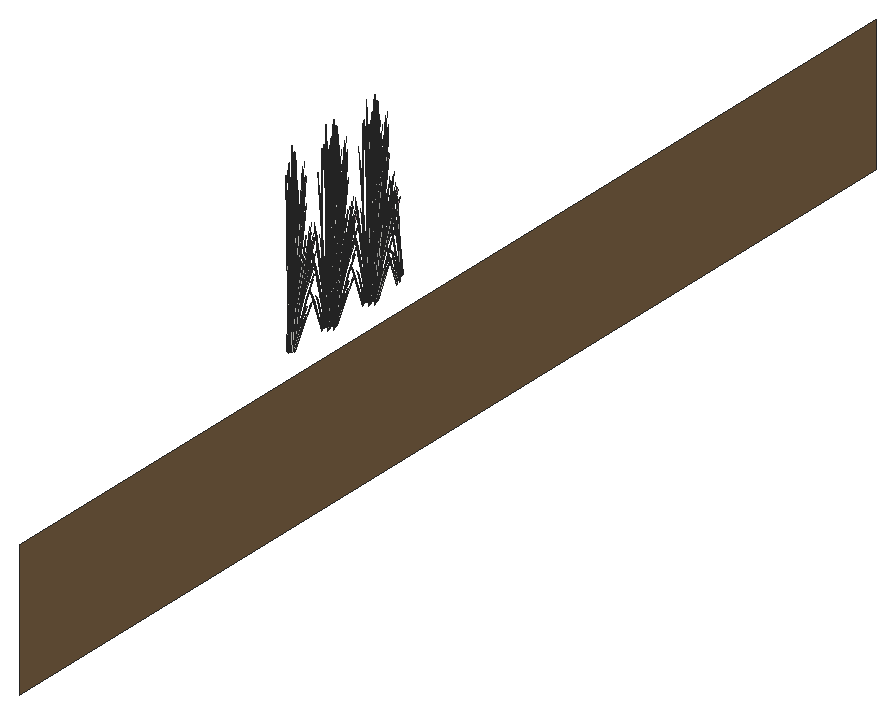
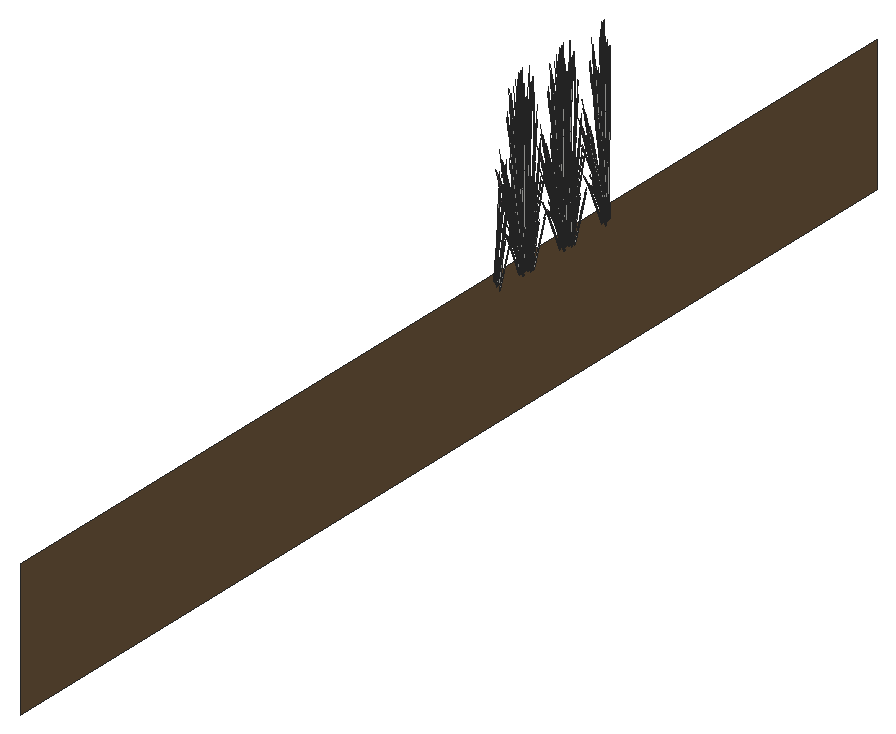
# SketchUp Ruby script. Lengths in inches.
U = 1.inch
M = Sketchup.active_model
def pt(a) = Geom::Point3d.new(a.map { |v| v * U })
def face(e, loops, mat)
  f = e.add_face(loops[0].map { |a| pt(a) })
  loops[1..].each { |l| e.add_face(l.map { |a| pt(a) }).erase! }
  f.material = f.back_material = mat if mat
  f
end
# faces: each face lists its corners as indices into pts; further lists are holes
def faces(e, pts, list, mat = nil) = list.each { |f| face(e, (f[0].is_a?(Array) ? f : [f]).map { |l| l.map { |i| pts[i] } }, mat) }
# xy, xz, yz: faces in a plane at the given z, y or x. An outline is a flat list of corners, or four numbers for a rectangle; further outlines are holes
def ring(l) = l.size == 4 ? [[l[0], l[1]], [l[2], l[1]], [l[2], l[3]], [l[0], l[3]]] : l.each_slice(2).to_a
def flat(e, list, mat, &to3) = list.each { |f| face(e, (f[0].is_a?(Array) ? f : [f]).map { |l| ring(l).map { |u, v| to3.(u, v) } }, mat) }
def xy(e, z, list, mat = nil) = flat(e, list, mat) { |x, y| [x, y, z] }
def xz(e, y, list, mat = nil) = flat(e, list, mat) { |x, z| [x, y, z] }
def yz(e, x, list, mat = nil) = flat(e, list, mat) { |y, z| [x, y, z] }
def lines(e, pts, list) = list.each { |a, b| e.add_line(pt(pts[a]), pt(pts[b])) }
# prism: a flat outline (further loops are holes) pulled along v
def prism(e, loops, v, mat = nil)
  f = face(e, loops, mat); d = Geom::Vector3d.new(v.map { |x| x * U })
  f.pushpull(f.normal.samedirection?(d) ? d.length : -d.length)
end
def box(e, o, s, mat = nil) = prism(e, [[o, [o[0] + s[0], o[1], o[2]], [o[0] + s[0], o[1] + s[1], o[2]], [o[0], o[1] + s[1], o[2]]]], [0, 0, s[2]], mat)
def at(x, y, z, deg = 0) = Geom::Transformation.translation(pt([x, y, z])) * Geom::Transformation.rotation(ORIGIN, Z_AXIS, deg.degrees)
def axes(o, x, y, z) = Geom::Transformation.new([*x, 0, *y, 0, *z, 0, *pt(o).to_a, 1])
def part(name) = M.definitions.add(name)
# library, detail: a bought-in or finely detailed component or shape, given as its bounding box
def library(name, o, s) = part(name).tap { |d| box(d.entities, o, s) }
def detail(e, o, s) = box(e.add_group.entities, o, s)
def put(e, d, t, mat = nil) = e.add_instance(d, t).tap { |i| i.material = mat if mat }
def group(e, t, mat = nil) = e.add_group.tap { |g| g.transformation = t; g.material = mat if mat }.entities
root = M.entities
M.materials.add("LightPink_Translucent").color = [144, 107, 117]
M.materials["LightPink_Translucent"].alpha = 0.75
M.materials.add("Soil_03_1K").color = [122, 96, 67]
c1 = part("blade")
p = [[2.15,0.21,22],[0,0.17,0],[0.09,0.45,0],[2.18,0.31,22],[2.29,0.31,22],[0.38,0.45,0],
  [2.48,0.24,33],[2.49,0.24,33],[2.48,0.22,33]]
faces(c1.entities,p,[[0,1,2,3],[4,5,2,3],[6,3,4,7],[8,0,3,6]])
c2 = part("seeds")
p = [[0.3,-0.1,1.38],[-0.01,-0.03,1.59],[-0.01,-0.03,0.03],[0.14,-0.07,-0.07],[0.29,-0.03,3],[0.15,0.01,3.11]]
faces(c2.entities,p,[[0,1,2,3],[1,0,4,5]],"LightPink_Translucent")
c3 = part("blade with seeds")
put(c3.entities,c1,at(0,0,0))
put(c3.entities,c2,axes([2.4,0.25,30.99],[1.5799,-0.05474,1.17369],[-0.12525,1.92788,0.29478],[-0.07173,-0.02425,1.56792]))
yz(root,410.57,[[509.26,-48,890.67,0]],"Soil_03_1K")
put(root,c3,axes([402.5,638.32,2.38],[-0.44609,-0.09826,0.49198],[0.09078,-0.55493,0.19306],[0.06519,0.05359,1.70813]))
put(root,c3,axes([402.15,639.6875,2.2],[-0.11516,-0.40207,0],[0.32884,-0.1408,0],[0,0,1.54371]))
put(root,c3,axes([402.58,639.63,2.18],[0.37054,-0.15823,-0.19198],[0.1302,0.45581,0.00008],[0.0409,-0.01749,1.73897]))
put(root,c3,axes([402.62,638.77,2.21],[0.24637,0.30123,0],[-0.24637,0.30123,0],[0,0,1.69266]))
put(root,c3,axes([403.29,638.64,2.47],[-0.2773,-0.3397,0.17642],[0.27945,-0.32949,0.35086],[-0.03063,0.06937,1.60407]))
put(root,c3,axes([402.78,638.125,2.06],[0.36714,0.07646,-0.62353],[-0.07747,0.47163,-0.16365],[0.10956,0.05715,1.37633]))
put(root,c3,axes([404.4,638.95,2.77],[-0.21807,0.07699,1.1486],[0.10265,-0.31819,0.84392],[0.11568,0.02177,0.25299]))
put(root,c3,axes([402.62,638.42,2.72],[0.17124,-0.42022,0.44739],[0.35581,0.20224,-0.21531],[0,0.09687,1.43643]))
put(root,c3,axes([402.55,638.66,2.29],[0,0.53934,-0.05637],[-0.44133,0,0],[0,0.01695,1.79368]))
put(root,c3,axes([402.58,638.28,2.21],[0.21202,0.39143,-0.44739],[-0.32115,0.27564,0.21531],[0.06861,0.04843,1.43643]))
put(root,c3,axes([404.02,639.93,3.93],[-0.06755,-0.39203,-0.03492],[0.31928,-0.09013,-0.15832],[0.06667,0.02485,0.52218]))
put(root,c3,axes([403.52,638.65,2.48],[0,-0.46636,0.49651],[0.39487,0,0],[0,0.10622,1.57504]))
put(root,c3,axes([402.77,638.51,2.62],[0.32884,-0.136,0.1448],[0.11516,0.38837,-0.41347],[0,0.08547,1.26744]))
put(root,c3,axes([403.99,639.46,2.59],[-0.085,-0.1147,1.43002],[0.1106,-0.37943,-0.30754],[0.17198,0.0514,0.61141]))
put(root,c3,axes([402.47,639.88,2.2],[0.35581,0.20937,0],[-0.17124,0.43505,0],[0,0,1.74954]))
put(root,c3,axes([403.21,639.69,4.98],[0.35281,0.01123,-0.71045],[-0.0237,0.47284,0.08574],[0.14947,0.0499,1.00501]))
put(root,c3,axes([402.8125,640.07,2.48],[0.33032,-0.23318,0.49651],[0.19744,0.41812,0],[-0.07523,0.05311,1.57504]))
put(root,c3,axes([402.34,639.7,2.29],[0.15345,0.53576,-0.06012],[-0.43845,0.18773,0],[0.00536,0.01871,1.72173]))
put(root,c3,axes([403.78,638.73,2.375],[0.44133,0,0],[0,0.52122,-0.51607],[0,0.11871,1.63711]))
put(root,c3,axes([403.61,639,2.2],[-0.44111,-0.00373,-0.04976],[0,-0.52122,0.49943],[-0.01386,0.11865,1.58352]))
put(root,c3,axes([402.65,638.55,2.67],[0.39748,0.22252,-0.29095],[-0.19139,0.46966,-0.50002],[0.01249,0.11531,1.59708]))
put(root,c3,axes([403.42,639.89,4.53],[0.20082,0.29199,-0.35414],[-0.2293,0.2764,0.4572],[0.1165,0.04206,0.87481]))
put(root,c3,axes([403.52,639.08,2.03],[-0.24637,0.29097,-0.30978],[-0.24637,-0.29097,0.30978],[0,0.09372,1.38974]))
put(root,c3,axes([402.61,638.9,2.21],[-0.17124,0.42022,-0.44739],[-0.35581,-0.20224,0.21531],[0,0.09687,1.43643]))
put(root,c3,axes([402.62,640.1,2.33],[0.44186,0.15158,0.30756],[-0.11054,0.54181,-0.36492],[-0.07313,0.06781,1.64885]))
put(root,c3,axes([403.6875,639.09,2.02],[0,0.46636,-0.49651],[-0.39487,0,0],[0,0.10622,1.57504]))
put(root,c3,axes([402.7,639.14,3.875],[-0.1311,-0.08035,1.71376],[0.27131,-0.33708,0.13857],[0.16909,0.15206,0.73262]))
put(root,c3,axes([403.18,640.05,2.77],[-0.19872,-0.13409,1.1486],[0.2566,-0.13625,0.84392],[0.06921,0.11541,0.25299]))
put(root,c3,axes([403.24,640.55,1.49],[0.02571,-0.06733,1.76342],[0.32373,-0.19829,-0.26939],[0.09815,0.10263,0.30037]))
put(root,c3,axes([402.8125,639.02,2.09],[0.12941,0.42699,-0.69212],[-0.37279,0.15378,-0.18165],[0.0143,0.14459,1.52773]))
put(root,c3,axes([402.74,640.24,4.68],[0.34827,-0.11086,-0.51099],[0.06092,0.41983,-0.3958],[0.09354,0.12031,0.97773]))
put(root,c3,axes([403.22,640.66,2.67],[-0.22633,-0.01463,1.0506],[0.14947,-0.31064,0.58006],[0.08941,0.11036,0.8241]))
put(root,c3,axes([402.48,639.91,2.59],[0.00623,-0.15459,1.43002],[0.29764,-0.17268,-0.30754],[0.09188,0.18503,0.61141]))
put(root,c3,axes([401.73,640.54,1.49],[0.05712,-0.02538,1.76342],[0.34359,0.13968,-0.26939],[0.01005,0.15742,0.30037]))
put(root,c3,axes([401.96,640.43,4.68],[0.34695,0.11691,-0.51099],[-0.11892,0.40083,-0.3958],[0.03181,0.16138,0.97773]))
put(root,c3,axes([402.16,639.61,3.875],[-0.08068,-0.14973,1.71376],[0.3728,-0.12606,0.13857],[0.08426,0.23506,0.73262]))
put(root,c3,axes([401.8,640.68,4.53],[-0.1064,0.35863,-0.35414],[-0.31043,-0.1046,0.4572],[0.02846,0.14439,0.87481]))
put(root,c3,axes([401.84,640.36,4.98],[0.16845,0.3792,-0.71045],[-0.34676,0.21133,0.08574],[0.03939,0.18322,1.00501]))
put(root,c3,axes([402.72,655.13,2.59],[-0.10032,0.0944,1.43002],[-0.30046,-0.16522,-0.30754],[0.05569,-0.20547,0.61141]))
put(root,c3,axes([401.98,654.62,1.49],[-0.0592,0.0168,1.76342],[-0.32738,-0.18913,-0.26939],[0.00549,-0.15776,0.30037]))
put(root,c3,axes([402.97,655.83,4.98],[0.00918,-0.43138,-0.71045],[0.38672,0.02897,0.08574],[0.04081,-0.18275,1.00501]))
put(root,c3,axes([402.3,655.14,4.53],[0.1064,-0.35863,-0.35414],[0.31043,0.1046,0.4572],[-0.02846,-0.14439,0.87481]))
put(root,c3,axes([402.53,655.61,3.875],[-0.06572,0.16029,1.71376],[-0.27569,-0.33172,0.13857],[0.12437,-0.20675,0.73262]))
put(root,c3,axes([402.35,654.38,2.77],[0.04528,0.27194,1.1486],[-0.25117,-0.15062,0.84392],[0.02703,-0.13924,0.25299]))
put(root,c3,axes([402.89,655.6875,4.68],[-0.25266,-0.31335,-0.51099],[0.2669,-0.27442,-0.3958],[0.03844,-0.15921,0.97773]))
put(root,c3,axes([403.13,655.57,4.53],[0.23881,-0.24554,-0.35414],[0.22606,0.28036,0.4572],[0.0344,-0.14245,0.87481]))
put(root,c3,axes([403.43,655.42,1.49],[-0.05283,-0.03674,1.76342],[-0.13569,-0.41045,-0.26939],[0.09154,-0.11138,0.30037]))
put(root,c3,axes([403.42,656.58,4.98],[0.18436,-0.36797,-0.71045],[0.32306,0.26151,0.08574],[0.11008,-0.13332,1.00501]))
put(root,c3,axes([401.43,655.51,2.375],[-0.22066,-0.46731,0],[0.36918,-0.26061,-0.51607],[0.08408,-0.05936,1.63711]))
put(root,c3,axes([403.41,656.41,4.68],[-0.09067,-0.42583,-0.51099],[0.34336,-0.07449,-0.3958],[0.0984,-0.11438,0.97773]))
put(root,c3,axes([401.73,655.4375,2.02],[0.33032,-0.23318,-0.49651],[0.19744,0.41812,0],[0.07523,-0.05311,1.57504]))
put(root,c3,axes([403.69,656.24,2.59],[-0.12609,-0.01381,1.43002],[-0.12917,-0.37055,-0.30754],[0.1549,-0.10482,0.61141]))
put(root,c3,axes([402.12,656.39,2.06],[0.23773,-0.35053,-0.62353],[0.29532,0.31785,-0.16365],[0.09526,-0.08744,1.37633]))
put(root,c3,axes([403.84,655.5625,2.77],[-0.11756,0.2374,1.1486],[-0.10105,-0.31895,0.84392],[0.09709,-0.07992,0.25299]))
put(root,c3,axes([403.67,656.45,4.53],[0.30722,-0.06665,-0.35414],[0.08112,0.381,0.4572],[0.08804,-0.10234,0.87481]))
put(root,c3,axes([401.71,657.01,2.21],[0.17124,-0.42022,-0.44739],[0.35581,0.20224,0.21531],[0,-0.09687,1.43643]))
put(root,c3,axes([401.86,656.8,2.67],[-0.04113,-0.53214,-0.29095],[0.42835,-0.03218,-0.50002],[0.07543,-0.07088,1.59708]))
put(root,c3,axes([401.81,655.62,2.03],[0.32928,0.11539,-0.30978],[-0.08291,0.40636,0.30978],[0.06638,-0.04686,1.38974]))
put(root,c3,axes([401.92,657.22,2.43],[0.39767,0.22603,0.24065],[-0.19139,0.46966,0.50002],[0,-0.10827,1.60543]))
put(root,c3,axes([401.79,656.9,2.72],[-0.38326,0.02879,0.44739],[-0.03466,-0.47788,-0.21531],[0.06861,-0.04843,1.43643]))
put(root,c3,axes([403.57,657.35,4.68],[0.09562,-0.42421,-0.51099],[0.32782,0.1454,-0.3958],[0.13199,-0.0389,0.97773]))
put(root,c3,axes([403.06,655.625,2.375],[0.22066,-0.46731,0],[0.36918,0.26061,-0.51607],[0.08408,0.05936,1.63711]))
put(root,c3,axes([401.78,657.07,2.36],[0.15345,0.52148,0.45755],[-0.43845,0.18134,0.17955],[0.00536,-0.09582,1.58856]))
put(root,c3,axes([403.92,657.47,1.98],[-0.22732,0.05597,1.41583],[-0.03618,-0.44548,0.08104],[0.15921,-0.06743,0.80566]))
put(root,c3,axes([404.34,657.08,2.26],[-0.21881,-0.29821,-0.06488],[0.23965,-0.27324,-0.29416],[0.0679,-0.01924,0.97024]))
put(root,c3,axes([402.33,657.12,2.21],[0,-0.53961,0],[0.44133,0,0],[0,0,1.79456]))
put(root,c3,axes([402.87,655.87,2.48],[-0.33032,-0.23318,0.49651],[0.19744,-0.41812,0],[0.07523,0.05311,1.57504]))
put(root,c3,axes([403.51,657.51,4.98],[0.31014,-0.20596,-0.71045],[0.17284,0.42397,0.08574],[0.14985,-0.04816,1.00501]))
put(root,c3,axes([402.12,656.78,2.36],[-0.29264,0.42323,0.45755],[-0.34767,-0.3736,0.17955],[0.07055,-0.04224,1.58856]))
put(root,c3,axes([401.61,656.08,2.47],[-0.10196,0.46348,0.17642],[-0.3731,-0.13116,0.35086],[0.06445,-0.00226,1.60407]))
put(root,c3,axes([401.46,656.45,1.59],[-0.3474,0.18671,1.28929],[-0.11057,-0.53572,0.50096],[0.21332,0.00891,1.46642]))
put(root,c3,axes([402.39,656.6,2.62],[0.06809,-0.4162,0.1448],[0.33266,0.07225,-0.41347],[0.06054,0.04274,1.26744]))
put(root,c3,axes([404.17,657.18,1.49],[-0.01845,-0.0708,1.76342],[0.12793,-0.41416,-0.26939],[0.12905,-0.00596,0.30037]))
put(root,c3,axes([402.25,656.71,2.72],[-0.21202,-0.39143,0.44739],[0.32115,-0.27564,-0.21531],[0.06861,0.04843,1.43643]))
put(root,c3,axes([402.36,656.73,2.67],[0.35635,-0.30962,-0.29095],[0.23697,0.43749,-0.50002],[0.08792,0.04443,1.59708]))
put(root,c3,axes([403.78,657.55,4.53],[0.29332,0.1301,-0.35414],[-0.08555,0.37955,0.4572],[0.11809,-0.0348,0.87481]))
put(root,c3,axes([403.26,655.91,2.02],[0.33032,0.23318,-0.49651],[-0.19744,0.41812,0],[0.07523,0.05311,1.57504]))
put(root,c3,axes([402.63,657.24,2.21],[0.39487,0,0],[0,0.48281,0],[0,0,1.78407]))
put(root,c3,axes([402.74,656.11,2.47],[-0.37926,0.12378,0.17642],[-0.09365,-0.46065,0.35086],[0.03382,0.06712,1.60407]))
put(root,c3,axes([402.98,657.08,3.875],[-0.14639,0.01056,1.71376],[0.09712,-0.45778,0.13857],[0.20862,0.02831,0.73262]))
put(root,c3,axes([403.17,656.08,2.03],[0.08291,0.40636,-0.30978],[-0.32928,0.11539,0.30978],[0.06638,0.04686,1.38974]))
put(root,c3,axes([402.5,656.99,2.38],[-0.44609,-0.09826,0.49198],[0.09078,-0.55493,0.19306],[0.06519,0.05359,1.70813]))
put(root,c3,axes([402.15,658.36,2.2],[-0.11516,-0.40207,0],[0.32884,-0.1408,0],[0,0,1.54371]))
put(root,c3,axes([402.58,658.31,2.18],[0.37054,-0.15823,-0.19198],[0.1302,0.45581,0.00008],[0.0409,-0.01749,1.73897]))
put(root,c3,axes([402.62,657.44,2.21],[0.24637,0.30123,0],[-0.24637,0.30123,0],[0,0,1.69266]))
put(root,c3,axes([403.29,657.3125,2.47],[-0.2773,-0.3397,0.17642],[0.27945,-0.32949,0.35086],[-0.03063,0.06937,1.60407]))
put(root,c3,axes([402.78,656.8,2.06],[0.36714,0.07646,-0.62353],[-0.07747,0.47163,-0.16365],[0.10956,0.05715,1.37633]))
put(root,c3,axes([404.4,657.625,2.77],[-0.21807,0.07699,1.1486],[0.10265,-0.31819,0.84392],[0.11568,0.02177,0.25299]))
put(root,c3,axes([402.62,657.09,2.72],[0.17124,-0.42022,0.44739],[0.35581,0.20224,-0.21531],[0,0.09687,1.43643]))
put(root,c3,axes([402.55,657.33,2.29],[0,0.53934,-0.05637],[-0.44133,0,0],[0,0.01695,1.79368]))
put(root,c3,axes([402.58,656.95,2.21],[0.21202,0.39143,-0.44739],[-0.32115,0.27564,0.21531],[0.06861,0.04843,1.43643]))
put(root,c3,axes([404.02,658.61,3.93],[-0.06755,-0.39203,-0.03492],[0.31928,-0.09013,-0.15832],[0.06667,0.02485,0.52218]))
put(root,c3,axes([403.52,657.33,2.48],[0,-0.46636,0.49651],[0.39487,0,0],[0,0.10622,1.57504]))
put(root,c3,axes([402.77,657.1875,2.62],[0.32884,-0.136,0.1448],[0.11516,0.38837,-0.41347],[0,0.08547,1.26744]))
put(root,c3,axes([403.99,658.13,2.59],[-0.085,-0.1147,1.43002],[0.1106,-0.37943,-0.30754],[0.17198,0.0514,0.61141]))
put(root,c3,axes([402.47,658.55,2.2],[0.35581,0.20937,0],[-0.17124,0.43505,0],[0,0,1.74954]))
put(root,c3,axes([403.21,658.37,4.98],[0.35281,0.01123,-0.71045],[-0.0237,0.47284,0.08574],[0.14947,0.0499,1.00501]))
put(root,c3,axes([402.8125,658.74,2.48],[0.33032,-0.23318,0.49651],[0.19744,0.41812,0],[-0.07523,0.05311,1.57504]))
put(root,c3,axes([402.34,658.375,2.29],[0.15345,0.53576,-0.06012],[-0.43845,0.18773,0],[0.00536,0.01871,1.72173]))
put(root,c3,axes([403.78,657.41,2.375],[0.44133,0,0],[0,0.52122,-0.51607],[0,0.11871,1.63711]))
put(root,c3,axes([403.61,657.67,2.2],[-0.44111,-0.00373,-0.04976],[0,-0.52122,0.49943],[-0.01386,0.11865,1.58352]))
put(root,c3,axes([402.65,657.22,2.67],[0.39748,0.22252,-0.29095],[-0.19139,0.46966,-0.50002],[0.01249,0.11531,1.59708]))
put(root,c3,axes([403.42,658.56,4.53],[0.20082,0.29199,-0.35414],[-0.2293,0.2764,0.4572],[0.1165,0.04206,0.87481]))
put(root,c3,axes([403.52,657.75,2.03],[-0.24637,0.29097,-0.30978],[-0.24637,-0.29097,0.30978],[0,0.09372,1.38974]))
put(root,c3,axes([402.61,657.57,2.21],[-0.17124,0.42022,-0.44739],[-0.35581,-0.20224,0.21531],[0,0.09687,1.43643]))
put(root,c3,axes([402.62,658.77,2.33],[0.44186,0.15158,0.30756],[-0.11054,0.54181,-0.36492],[-0.07313,0.06781,1.64885]))
put(root,c3,axes([403.6875,657.76,2.02],[0,0.46636,-0.49651],[-0.39487,0,0],[0,0.10622,1.57504]))
put(root,c3,axes([402.7,657.8125,3.875],[-0.1311,-0.08035,1.71376],[0.27131,-0.33708,0.13857],[0.16909,0.15206,0.73262]))
put(root,c3,axes([403.18,658.73,2.77],[-0.19872,-0.13409,1.1486],[0.2566,-0.13625,0.84392],[0.06921,0.11541,0.25299]))
put(root,c3,axes([403.24,659.22,1.49],[0.02571,-0.06733,1.76342],[0.32373,-0.19829,-0.26939],[0.09815,0.10263,0.30037]))
put(root,c3,axes([402.8125,657.7,2.09],[0.12941,0.42699,-0.69212],[-0.37279,0.15378,-0.18165],[0.0143,0.14459,1.52773]))
put(root,c3,axes([402.74,658.91,4.68],[0.34827,-0.11086,-0.51099],[0.06092,0.41983,-0.3958],[0.09354,0.12031,0.97773]))
put(root,c3,axes([403.22,659.34,2.67],[-0.22633,-0.01463,1.0506],[0.14947,-0.31064,0.58006],[0.08941,0.11036,0.8241]))
put(root,c3,axes([402.48,658.58,2.59],[0.00623,-0.15459,1.43002],[0.29764,-0.17268,-0.30754],[0.09188,0.18503,0.61141]))
put(root,c3,axes([401.73,659.21,1.49],[0.05712,-0.02538,1.76342],[0.34359,0.13968,-0.26939],[0.01005,0.15742,0.30037]))
put(root,c3,axes([401.96,659.11,4.68],[0.34695,0.11691,-0.51099],[-0.11892,0.40083,-0.3958],[0.03181,0.16138,0.97773]))
put(root,c3,axes([402.16,658.28,3.875],[-0.08068,-0.14973,1.71376],[0.3728,-0.12606,0.13857],[0.08426,0.23506,0.73262]))
put(root,c3,axes([401.8,659.35,4.53],[-0.1064,0.35863,-0.35414],[-0.31043,-0.1046,0.4572],[0.02846,0.14439,0.87481]))
put(root,c3,axes([401.84,659.03,4.98],[0.16845,0.3792,-0.71045],[-0.34676,0.21133,0.08574],[0.03939,0.18322,1.00501]))
put(root,c3,axes([402.72,673.35,2.59],[-0.10032,0.0944,1.43002],[-0.30046,-0.16522,-0.30754],[0.05569,-0.20547,0.61141]))
put(root,c3,axes([401.98,672.83,1.49],[-0.0592,0.0168,1.76342],[-0.32738,-0.18913,-0.26939],[0.00549,-0.15776,0.30037]))
put(root,c3,axes([402.97,674.05,4.98],[0.00918,-0.43138,-0.71045],[0.38672,0.02897,0.08574],[0.04081,-0.18275,1.00501]))
put(root,c3,axes([402.3,673.35,4.53],[0.1064,-0.35863,-0.35414],[0.31043,0.1046,0.4572],[-0.02846,-0.14439,0.87481]))
put(root,c3,axes([402.53,673.83,3.875],[-0.06572,0.16029,1.71376],[-0.27569,-0.33172,0.13857],[0.12437,-0.20675,0.73262]))
put(root,c3,axes([402.35,672.59,2.77],[0.04528,0.27194,1.1486],[-0.25117,-0.15062,0.84392],[0.02703,-0.13924,0.25299]))
put(root,c3,axes([402.89,673.9,4.68],[-0.25266,-0.31335,-0.51099],[0.2669,-0.27442,-0.3958],[0.03844,-0.15921,0.97773]))
put(root,c3,axes([403.13,673.79,4.53],[0.23881,-0.24554,-0.35414],[0.22606,0.28036,0.4572],[0.0344,-0.14245,0.87481]))
put(root,c3,axes([403.43,673.64,1.49],[-0.05283,-0.03674,1.76342],[-0.13569,-0.41045,-0.26939],[0.09154,-0.11138,0.30037]))
put(root,c3,axes([403.42,674.8,4.98],[0.18436,-0.36797,-0.71045],[0.32306,0.26151,0.08574],[0.11008,-0.13332,1.00501]))
put(root,c3,axes([401.43,673.72,2.375],[-0.22066,-0.46731,0],[0.36918,-0.26061,-0.51607],[0.08408,-0.05936,1.63711]))
put(root,c3,axes([403.41,674.625,4.68],[-0.09067,-0.42583,-0.51099],[0.34336,-0.07449,-0.3958],[0.0984,-0.11438,0.97773]))
put(root,c3,axes([401.73,673.65,2.02],[0.33032,-0.23318,-0.49651],[0.19744,0.41812,0],[0.07523,-0.05311,1.57504]))
put(root,c3,axes([403.69,674.46,2.59],[-0.12609,-0.01381,1.43002],[-0.12917,-0.37055,-0.30754],[0.1549,-0.10482,0.61141]))
put(root,c3,axes([402.12,674.61,2.06],[0.23773,-0.35053,-0.62353],[0.29532,0.31785,-0.16365],[0.09526,-0.08744,1.37633]))
put(root,c3,axes([403.84,673.78,2.77],[-0.11756,0.2374,1.1486],[-0.10105,-0.31895,0.84392],[0.09709,-0.07992,0.25299]))
put(root,c3,axes([403.67,674.67,4.53],[0.30722,-0.06665,-0.35414],[0.08112,0.381,0.4572],[0.08804,-0.10234,0.87481]))
put(root,c3,axes([401.71,675.22,2.21],[0.17124,-0.42022,-0.44739],[0.35581,0.20224,0.21531],[0,-0.09687,1.43643]))
put(root,c3,axes([401.86,675.01,2.67],[-0.04113,-0.53214,-0.29095],[0.42835,-0.03218,-0.50002],[0.07543,-0.07088,1.59708]))
put(root,c3,axes([401.81,673.84,2.03],[0.32928,0.11539,-0.30978],[-0.08291,0.40636,0.30978],[0.06638,-0.04686,1.38974]))
put(root,c3,axes([401.92,675.43,2.43],[0.39767,0.22603,0.24065],[-0.19139,0.46966,0.50002],[0,-0.10827,1.60543]))
put(root,c3,axes([401.79,675.12,2.72],[-0.38326,0.02879,0.44739],[-0.03466,-0.47788,-0.21531],[0.06861,-0.04843,1.43643]))
put(root,c3,axes([403.57,675.57,4.68],[0.09562,-0.42421,-0.51099],[0.32782,0.1454,-0.3958],[0.13199,-0.0389,0.97773]))
put(root,c3,axes([403.06,673.84,2.375],[0.22066,-0.46731,0],[0.36918,0.26061,-0.51607],[0.08408,0.05936,1.63711]))
put(root,c3,axes([401.78,675.29,2.36],[0.15345,0.52148,0.45755],[-0.43845,0.18134,0.17955],[0.00536,-0.09582,1.58856]))
put(root,c3,axes([403.92,675.6875,1.98],[-0.22732,0.05597,1.41583],[-0.03618,-0.44548,0.08104],[0.15921,-0.06743,0.80566]))
put(root,c3,axes([404.34,675.29,2.26],[-0.21881,-0.29821,-0.06488],[0.23965,-0.27324,-0.29416],[0.0679,-0.01924,0.97024]))
put(root,c3,axes([402.33,675.33,2.21],[0,-0.53961,0],[0.44133,0,0],[0,0,1.79456]))
put(root,c3,axes([402.87,674.09,2.48],[-0.33032,-0.23318,0.49651],[0.19744,-0.41812,0],[0.07523,0.05311,1.57504]))
put(root,c3,axes([403.51,675.72,4.98],[0.31014,-0.20596,-0.71045],[0.17284,0.42397,0.08574],[0.14985,-0.04816,1.00501]))
put(root,c3,axes([402.12,674.99,2.36],[-0.29264,0.42323,0.45755],[-0.34767,-0.3736,0.17955],[0.07055,-0.04224,1.58856]))
put(root,c3,axes([401.61,674.3,2.47],[-0.10196,0.46348,0.17642],[-0.3731,-0.13116,0.35086],[0.06445,-0.00226,1.60407]))
put(root,c3,axes([401.46,674.67,1.59],[-0.3474,0.18671,1.28929],[-0.11057,-0.53572,0.50096],[0.21332,0.00891,1.46642]))
put(root,c3,axes([402.39,674.8125,2.62],[0.06809,-0.4162,0.1448],[0.33266,0.07225,-0.41347],[0.06054,0.04274,1.26744]))
put(root,c3,axes([404.17,675.4,1.49],[-0.01845,-0.0708,1.76342],[0.12793,-0.41416,-0.26939],[0.12905,-0.00596,0.30037]))
put(root,c3,axes([402.25,674.92,2.72],[-0.21202,-0.39143,0.44739],[0.32115,-0.27564,-0.21531],[0.06861,0.04843,1.43643]))
put(root,c3,axes([402.36,674.95,2.67],[0.35635,-0.30962,-0.29095],[0.23697,0.43749,-0.50002],[0.08792,0.04443,1.59708]))
put(root,c3,axes([403.78,675.76,4.53],[0.29332,0.1301,-0.35414],[-0.08555,0.37955,0.4572],[0.11809,-0.0348,0.87481]))
put(root,c3,axes([403.26,674.12,2.02],[0.33032,0.23318,-0.49651],[-0.19744,0.41812,0],[0.07523,0.05311,1.57504]))
put(root,c3,axes([402.63,675.45,2.21],[0.39487,0,0],[0,0.48281,0],[0,0,1.78407]))
put(root,c3,axes([402.74,674.32,2.47],[-0.37926,0.12378,0.17642],[-0.09365,-0.46065,0.35086],[0.03382,0.06712,1.60407]))
put(root,c3,axes([402.98,675.29,3.875],[-0.14639,0.01056,1.71376],[0.09712,-0.45778,0.13857],[0.20862,0.02831,0.73262]))
put(root,c3,axes([403.17,674.3,2.03],[0.08291,0.40636,-0.30978],[-0.32928,0.11539,0.30978],[0.06638,0.04686,1.38974]))
put(root,c3,axes([402.5,675.21,2.38],[-0.44609,-0.09826,0.49198],[0.09078,-0.55493,0.19306],[0.06519,0.05359,1.70813]))
put(root,c3,axes([402.15,676.58,2.2],[-0.11516,-0.40207,0],[0.32884,-0.1408,0],[0,0,1.54371]))
put(root,c3,axes([402.58,676.52,2.18],[0.37054,-0.15823,-0.19198],[0.1302,0.45581,0.00008],[0.0409,-0.01749,1.73897]))
put(root,c3,axes([402.62,675.66,2.21],[0.24637,0.30123,0],[-0.24637,0.30123,0],[0,0,1.69266]))
put(root,c3,axes([403.29,675.53,2.47],[-0.2773,-0.3397,0.17642],[0.27945,-0.32949,0.35086],[-0.03063,0.06937,1.60407]))
put(root,c3,axes([402.78,675.02,2.06],[0.36714,0.07646,-0.62353],[-0.07747,0.47163,-0.16365],[0.10956,0.05715,1.37633]))
put(root,c3,axes([404.4,675.84,2.77],[-0.21807,0.07699,1.1486],[0.10265,-0.31819,0.84392],[0.11568,0.02177,0.25299]))
put(root,c3,axes([402.62,675.31,2.72],[0.17124,-0.42022,0.44739],[0.35581,0.20224,-0.21531],[0,0.09687,1.43643]))
put(root,c3,axes([402.55,675.55,2.29],[0,0.53934,-0.05637],[-0.44133,0,0],[0,0.01695,1.79368]))
put(root,c3,axes([402.58,675.17,2.21],[0.21202,0.39143,-0.44739],[-0.32115,0.27564,0.21531],[0.06861,0.04843,1.43643]))
put(root,c3,axes([404.02,676.82,3.93],[-0.06755,-0.39203,-0.03492],[0.31928,-0.09013,-0.15832],[0.06667,0.02485,0.52218]))
put(root,c3,axes([403.52,675.54,2.48],[0,-0.46636,0.49651],[0.39487,0,0],[0,0.10622,1.57504]))
put(root,c3,axes([402.53,675.89,2.72],[0.38326,-0.02879,0.44739],[0.03466,0.47788,-0.21531],[-0.06861,0.04843,1.43643]))
put(root,c3,axes([402.77,675.4,2.62],[0.32884,-0.136,0.1448],[0.11516,0.38837,-0.41347],[0,0.08547,1.26744]))
put(root,c3,axes([403.99,676.35,2.59],[-0.085,-0.1147,1.43002],[0.1106,-0.37943,-0.30754],[0.17198,0.0514,0.61141]))
put(root,c3,axes([402.47,676.77,2.2],[0.35581,0.20937,0],[-0.17124,0.43505,0],[0,0,1.74954]))
put(root,c3,axes([403.21,676.58,4.98],[0.35281,0.01123,-0.71045],[-0.0237,0.47284,0.08574],[0.14947,0.0499,1.00501]))
put(root,c3,axes([402.8125,676.96,2.48],[0.33032,-0.23318,0.49651],[0.19744,0.41812,0],[-0.07523,0.05311,1.57504]))
put(root,c3,axes([402.34,676.59,2.29],[0.15345,0.53576,-0.06012],[-0.43845,0.18773,0],[0.00536,0.01871,1.72173]))
put(root,c3,axes([403.78,675.62,2.375],[0.44133,0,0],[0,0.52122,-0.51607],[0,0.11871,1.63711]))
put(root,c3,axes([403.61,675.89,2.2],[-0.44111,-0.00373,-0.04976],[0,-0.52122,0.49943],[-0.01386,0.11865,1.58352]))
put(root,c3,axes([402.65,675.44,2.67],[0.39748,0.22252,-0.29095],[-0.19139,0.46966,-0.50002],[0.01249,0.11531,1.59708]))
put(root,c3,axes([403.42,676.78,4.53],[0.20082,0.29199,-0.35414],[-0.2293,0.2764,0.4572],[0.1165,0.04206,0.87481]))
put(root,c3,axes([403.52,675.96,2.03],[-0.24637,0.29097,-0.30978],[-0.24637,-0.29097,0.30978],[0,0.09372,1.38974]))
put(root,c3,axes([402.61,675.78,2.21],[-0.17124,0.42022,-0.44739],[-0.35581,-0.20224,0.21531],[0,0.09687,1.43643]))
put(root,c3,axes([402.62,676.99,2.33],[0.44186,0.15158,0.30756],[-0.11054,0.54181,-0.36492],[-0.07313,0.06781,1.64885]))
put(root,c3,axes([403.6875,675.97,2.02],[0,0.46636,-0.49651],[-0.39487,0,0],[0,0.10622,1.57504]))
put(root,c3,axes([402.7,676.03,3.875],[-0.1311,-0.08035,1.71376],[0.27131,-0.33708,0.13857],[0.16909,0.15206,0.73262]))
put(root,c3,axes([403.18,676.94,2.77],[-0.19872,-0.13409,1.1486],[0.2566,-0.13625,0.84392],[0.06921,0.11541,0.25299]))
put(root,c3,axes([403.24,677.44,1.49],[0.02571,-0.06733,1.76342],[0.32373,-0.19829,-0.26939],[0.09815,0.10263,0.30037]))
put(root,c3,axes([402.8125,675.91,2.09],[0.12941,0.42699,-0.69212],[-0.37279,0.15378,-0.18165],[0.0143,0.14459,1.52773]))
put(root,c3,axes([402.74,677.125,4.68],[0.34827,-0.11086,-0.51099],[0.06092,0.41983,-0.3958],[0.09354,0.12031,0.97773]))
put(root,c3,axes([403.22,677.55,2.67],[-0.22633,-0.01463,1.0506],[0.14947,-0.31064,0.58006],[0.08941,0.11036,0.8241]))
put(root,c3,axes([402.48,676.8,2.59],[0.00623,-0.15459,1.43002],[0.29764,-0.17268,-0.30754],[0.09188,0.18503,0.61141]))
put(root,c3,axes([401.73,677.43,1.49],[0.05712,-0.02538,1.76342],[0.34359,0.13968,-0.26939],[0.01005,0.15742,0.30037]))
put(root,c3,axes([401.96,677.32,4.68],[0.34695,0.11691,-0.51099],[-0.11892,0.40083,-0.3958],[0.03181,0.16138,0.97773]))
put(root,c3,axes([402.16,676.49,3.875],[-0.08068,-0.14973,1.71376],[0.3728,-0.12606,0.13857],[0.08426,0.23506,0.73262]))
put(root,c3,axes([401.8,677.57,4.53],[-0.1064,0.35863,-0.35414],[-0.31043,-0.1046,0.4572],[0.02846,0.14439,0.87481]))
put(root,c3,axes([401.84,677.25,4.98],[0.16845,0.3792,-0.71045],[-0.34676,0.21133,0.08574],[0.03939,0.18322,1.00501]))
put(root,c3,axes([402.72,688.42,2.59],[-0.10032,0.0944,1.43002],[-0.30046,-0.16522,-0.30754],[0.05569,-0.20547,0.61141]))
put(root,c3,axes([401.98,687.91,1.49],[-0.0592,0.0168,1.76342],[-0.32738,-0.18913,-0.26939],[0.00549,-0.15776,0.30037]))
put(root,c3,axes([402.97,689.12,4.98],[0.00918,-0.43138,-0.71045],[0.38672,0.02897,0.08574],[0.04081,-0.18275,1.00501]))
put(root,c3,axes([402.3,688.43,4.53],[0.1064,-0.35863,-0.35414],[0.31043,0.1046,0.4572],[-0.02846,-0.14439,0.87481]))
put(root,c3,axes([402.53,688.9,3.875],[-0.06572,0.16029,1.71376],[-0.27569,-0.33172,0.13857],[0.12437,-0.20675,0.73262]))
put(root,c3,axes([402.35,687.67,2.77],[0.04528,0.27194,1.1486],[-0.25117,-0.15062,0.84392],[0.02703,-0.13924,0.25299]))
put(root,c3,axes([402.89,688.98,4.68],[-0.25266,-0.31335,-0.51099],[0.2669,-0.27442,-0.3958],[0.03844,-0.15921,0.97773]))
put(root,c3,axes([403.13,688.86,4.53],[0.23881,-0.24554,-0.35414],[0.22606,0.28036,0.4572],[0.0344,-0.14245,0.87481]))
